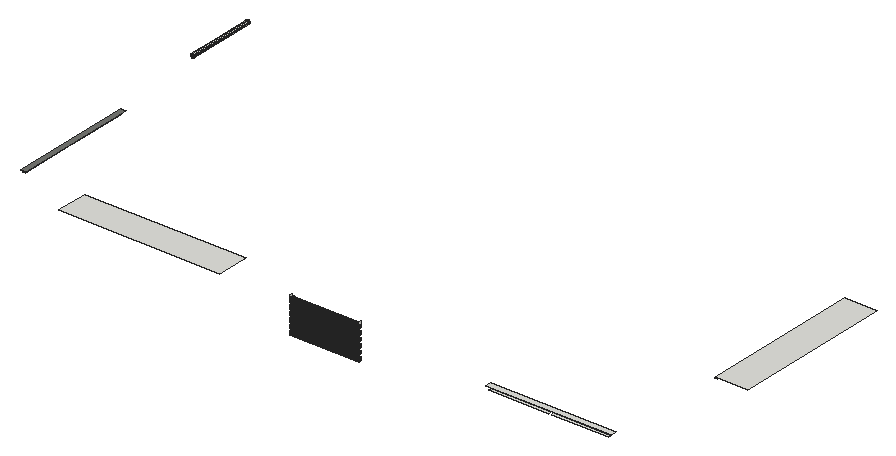
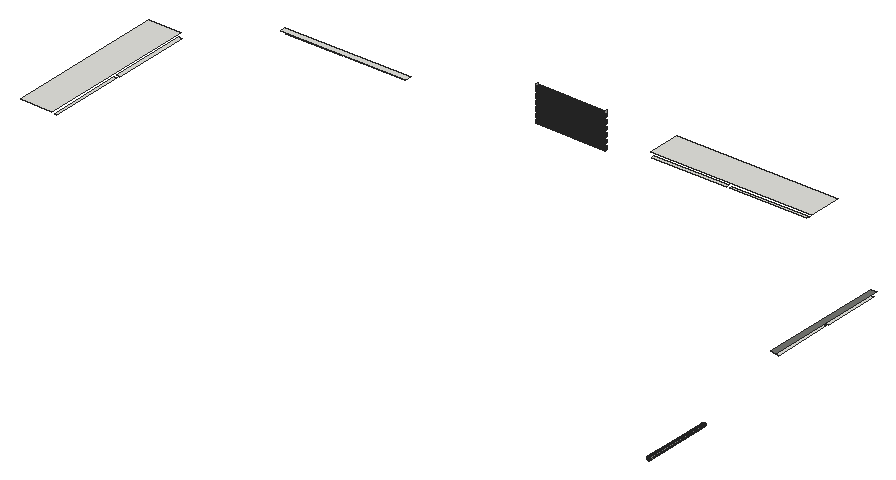
# SketchUp Ruby script. Lengths in inches.
U = 1.inch
M = Sketchup.active_model
def pt(a) = Geom::Point3d.new(a.map { |v| v * U })
def face(e, loops, mat)
  f = e.add_face(loops[0].map { |a| pt(a) })
  loops[1..].each { |l| e.add_face(l.map { |a| pt(a) }).erase! }
  f.material = f.back_material = mat if mat
  f
end
# faces: each face lists its corners as indices into pts; further lists are holes
def faces(e, pts, list, mat = nil) = list.each { |f| face(e, (f[0].is_a?(Array) ? f : [f]).map { |l| l.map { |i| pts[i] } }, mat) }
# xy, xz, yz: faces in a plane at the given z, y or x. An outline is a flat list of corners, or four numbers for a rectangle; further outlines are holes
def ring(l) = l.size == 4 ? [[l[0], l[1]], [l[2], l[1]], [l[2], l[3]], [l[0], l[3]]] : l.each_slice(2).to_a
def flat(e, list, mat, &to3) = list.each { |f| face(e, (f[0].is_a?(Array) ? f : [f]).map { |l| ring(l).map { |u, v| to3.(u, v) } }, mat) }
def xy(e, z, list, mat = nil) = flat(e, list, mat) { |x, y| [x, y, z] }
def xz(e, y, list, mat = nil) = flat(e, list, mat) { |x, z| [x, y, z] }
def yz(e, x, list, mat = nil) = flat(e, list, mat) { |y, z| [x, y, z] }
def lines(e, pts, list) = list.each { |a, b| e.add_line(pt(pts[a]), pt(pts[b])) }
# prism: a flat outline (further loops are holes) pulled along v
def prism(e, loops, v, mat = nil)
  f = face(e, loops, mat); d = Geom::Vector3d.new(v.map { |x| x * U })
  f.pushpull(f.normal.samedirection?(d) ? d.length : -d.length)
end
def box(e, o, s, mat = nil) = prism(e, [[o, [o[0] + s[0], o[1], o[2]], [o[0] + s[0], o[1] + s[1], o[2]], [o[0], o[1] + s[1], o[2]]]], [0, 0, s[2]], mat)
def at(x, y, z, deg = 0) = Geom::Transformation.translation(pt([x, y, z])) * Geom::Transformation.rotation(ORIGIN, Z_AXIS, deg.degrees)
def axes(o, x, y, z) = Geom::Transformation.new([*x, 0, *y, 0, *z, 0, *pt(o).to_a, 1])
def part(name) = M.definitions.add(name)
# library, detail: a bought-in or finely detailed component or shape, given as its bounding box
def library(name, o, s) = part(name).tap { |d| box(d.entities, o, s) }
def detail(e, o, s) = box(e.add_group.entities, o, s)
def put(e, d, t, mat = nil) = e.add_instance(d, t).tap { |i| i.material = mat if mat }
def group(e, t, mat = nil) = e.add_group.tap { |g| g.transformation = t; g.material = mat if mat }.entities
root = M.entities
M.materials.add("[Metal Seamed]").color = [118, 119, 115]
xy(root,647.61,[[1161.2,84.8125,1285.04,90.8125],[1291.04,84.8125,1408.89,90.8125],[120,175.92,126,293.77],[120,299.77,126,423.61]])
xy(root,653.61,[[1155.2,84.8125,1414.89,96.8125]])
xy(root,653.61,[[120,169.92,132,429.61]],"[Metal Seamed]")
xy(root,696.625,[[312.65,102.8125,473.9375,108.8125],[479.9375,102.8125,635.22,108.8125],[1476,277.47,1482,438.75],[1476,444.75,1482,600.03]])
xy(root,702.625,[[306.65,36.8125,641.22,102.8125],[1482,271.47,1548,606.03]])
yz(root,778.64,[[48.34,702.02,49.29,702.14,50.18,702.51,50.95,703.1,51.53,703.86,51.9,704.75,52.03,705.7,51.9,706.66,51.8,706.89,44.875,706.89,44.78,706.66,44.65,705.7,44.78,704.75,45.15,703.86,45.73,703.1,46.5,702.51,47.38,702.14]])
yz(root,922.01,[[48.34,702.02,47.38,702.14,46.5,702.51,45.73,703.1,45.15,703.86,44.78,704.75,44.65,705.7,44.78,706.66,44.875,706.89,51.8,706.89,51.9,706.66,52.03,705.7,51.9,704.75,51.53,703.86,50.95,703.1,50.18,702.51,49.29,702.14]])
p = [[922.01,48.34,633.02],[922.01,47.38,633.14],[778.64,47.38,633.14],[778.64,48.34,633.02],[922.01,49.29,633.14],[778.64,49.29,633.14],
  [83.53,662.8,633.02],[82.57,662.8,633.14],[82.57,806.17,633.14],[83.53,806.17,633.02],[84.48,662.8,633.14],[84.48,806.17,633.14],
  [922.01,46.5,633.51],[778.64,46.5,633.51],[922.01,50.18,633.51],[778.64,50.18,633.51],[81.68,662.8,633.51],[81.68,806.17,633.51],
  [85.37,662.8,633.51],[85.37,806.17,633.51],[922.01,45.73,634.1],[778.64,45.73,634.1],[922.01,50.95,634.1],[778.64,50.95,634.1],
  [80.92,662.8,634.1],[80.92,806.17,634.1],[86.13,662.8,634.1],[86.13,806.17,634.1],[922.01,45.15,634.86],[778.64,45.15,634.86],
  [922.01,51.53,634.86],[778.64,51.53,634.86],[80.33,662.8,634.86],[80.33,806.17,634.86],[86.72,662.8,634.86],[86.72,806.17,634.86],
  [922.01,44.78,635.75],[778.64,44.78,635.75],[922.01,51.9,635.75],[778.64,51.9,635.75],[79.97,662.8,635.75],[79.97,806.17,635.75],
  [87.09,662.8,635.75],[87.09,806.17,635.75],[922.01,44.65,636.7],[778.64,44.65,636.7],[922.01,52.03,636.7],[778.64,52.03,636.7],
  [79.84,662.8,636.7],[79.84,806.17,636.7],[87.21,662.8,636.7],[87.21,806.17,636.7],[922.01,44.78,637.66],[778.64,44.78,637.66],
  [922.01,51.9,637.66],[778.64,51.9,637.66],[79.97,662.8,637.66],[79.97,806.17,637.66],[87.09,662.8,637.66],[87.09,806.17,637.66],
  [922.01,45.15,638.55],[778.64,45.15,638.55],[922.01,51.53,638.55],[778.64,51.53,638.55],[80.33,662.8,638.55],[80.33,806.17,638.55],
  [86.72,662.8,638.55],[86.72,806.17,638.55],[922.01,45.73,639.3125],[778.64,45.73,639.3125],[922.01,50.95,639.3125],[778.64,50.95,639.3125],
  [80.92,662.8,639.3125],[80.92,806.17,639.3125],[86.13,662.8,639.3125],[86.13,806.17,639.3125],[922.01,46.5,639.9],[778.64,46.5,639.9],
  [922.01,50.18,639.9],[778.64,50.18,639.9],[81.68,662.8,639.9],[81.68,806.17,639.9],[85.37,662.8,639.9],[85.37,806.17,639.9],
  [922.01,47.38,640.27],[778.64,47.38,640.27],[922.01,49.29,640.27],[778.64,49.29,640.27],[82.57,662.8,640.27],[82.57,806.17,640.27],
  [84.48,662.8,640.27],[84.48,806.17,640.27],[922.01,48.34,640.39],[778.64,48.34,640.39],[83.53,662.8,640.39],[83.53,806.17,640.39],
  [922.01,48.34,645.02],[922.01,47.38,645.14],[778.64,47.38,645.14],[778.64,48.34,645.02],[922.01,49.29,645.14],[778.64,49.29,645.14],
  [922.01,46.5,645.51],[778.64,46.5,645.51],[922.01,50.18,645.51],[778.64,50.18,645.51],[922.01,45.73,646.1],[778.64,45.73,646.1],
  [922.01,50.95,646.1],[778.64,50.95,646.1],[922.01,45.15,646.86],[778.64,45.15,646.86],[922.01,51.53,646.86],[778.64,51.53,646.86],
  [922.01,44.78,647.75],[778.64,44.78,647.75],[922.01,51.9,647.75],[778.64,51.9,647.75],[922.01,44.65,648.7],[778.64,44.65,648.7],
  [922.01,52.03,648.7],[778.64,52.03,648.7],[922.01,44.78,649.66],[778.64,44.78,649.66],[922.01,51.9,649.66],[778.64,51.9,649.66],
  [922.01,45.15,650.55],[778.64,45.15,650.55],[922.01,51.53,650.55],[778.64,51.53,650.55],[922.01,45.73,651.3125],[778.64,45.73,651.3125],
  [922.01,50.95,651.3125],[778.64,50.95,651.3125],[922.01,46.5,651.9],[778.64,46.5,651.9],[922.01,50.18,651.9],[778.64,50.18,651.9],
  [922.01,47.38,652.27],[778.64,47.38,652.27],[922.01,49.29,652.27],[778.64,49.29,652.27],[922.01,48.34,652.39],[778.64,48.34,652.39],
  [922.01,48.34,657.02],[922.01,47.38,657.14],[778.64,47.38,657.14],[778.64,48.34,657.02],[922.01,49.29,657.14],[778.64,49.29,657.14],
  [922.01,46.5,657.51],[778.64,46.5,657.51],[922.01,50.18,657.51],[778.64,50.18,657.51],[922.01,45.73,658.1],[778.64,45.73,658.1],
  [922.01,50.95,658.1],[778.64,50.95,658.1],[922.01,45.15,658.86],[778.64,45.15,658.86],[922.01,51.53,658.86],[778.64,51.53,658.86],
  [922.01,44.78,659.75],[778.64,44.78,659.75],[922.01,51.9,659.75],[778.64,51.9,659.75],[922.01,44.65,660.7],[778.64,44.65,660.7],
  [922.01,52.03,660.7],[778.64,52.03,660.7],[922.01,44.78,661.66],[778.64,44.78,661.66],[922.01,51.9,661.66],[778.64,51.9,661.66],
  [922.01,45.15,662.55],[778.64,45.15,662.55],[922.01,51.53,662.55],[778.64,51.53,662.55],[922.01,45.73,663.3125],[778.64,45.73,663.3125],
  [922.01,50.95,663.3125],[778.64,50.95,663.3125],[922.01,46.5,663.9],[778.64,46.5,663.9],[922.01,50.18,663.9],[778.64,50.18,663.9],
  [922.01,47.38,664.27],[778.64,47.38,664.27],[922.01,49.29,664.27],[778.64,49.29,664.27],[922.01,48.34,664.39],[778.64,48.34,664.39],
  [922.01,48.34,669.02],[922.01,47.38,669.14],[778.64,47.38,669.14],[778.64,48.34,669.02],[922.01,49.29,669.14],[778.64,49.29,669.14],
  [922.01,46.5,669.51],[778.64,46.5,669.51],[922.01,50.18,669.51],[778.64,50.18,669.51],[922.01,45.73,670.1],[778.64,45.73,670.1],
  [922.01,50.95,670.1],[778.64,50.95,670.1],[922.01,45.15,670.86],[778.64,45.15,670.86],[922.01,51.53,670.86],[778.64,51.53,670.86],
  [922.01,44.78,671.75],[778.64,44.78,671.75],[922.01,51.9,671.75],[778.64,51.9,671.75],[922.01,44.65,672.7],[778.64,44.65,672.7],
  [922.01,52.03,672.7],[778.64,52.03,672.7],[922.01,44.78,673.66],[778.64,44.78,673.66],[922.01,51.9,673.66],[778.64,51.9,673.66],
  [922.01,45.15,674.55],[778.64,45.15,674.55],[922.01,51.53,674.55],[778.64,51.53,674.55],[922.01,45.73,675.3125],[778.64,45.73,675.3125],
  [922.01,50.95,675.3125],[778.64,50.95,675.3125],[922.01,46.5,675.9],[778.64,46.5,675.9],[922.01,50.18,675.9],[778.64,50.18,675.9],
  [922.01,47.38,676.27],[778.64,47.38,676.27],[922.01,49.29,676.27],[778.64,49.29,676.27],[922.01,48.34,676.39],[778.64,48.34,676.39],
  [922.01,48.34,681.02],[922.01,47.38,681.14],[778.64,47.38,681.14],[778.64,48.34,681.02],[922.01,49.29,681.14],[778.64,49.29,681.14],
  [922.01,46.5,681.51],[778.64,46.5,681.51],[922.01,50.18,681.51],[778.64,50.18,681.51],[922.01,45.73,682.1],[778.64,45.73,682.1],
  [922.01,50.95,682.1],[778.64,50.95,682.1],[922.01,45.15,682.86],[778.64,45.15,682.86],[922.01,51.53,682.86],[778.64,51.53,682.86],
  [922.01,44.78,683.75],[778.64,44.78,683.75],[922.01,51.9,683.75],[778.64,51.9,683.75],[922.01,44.65,684.7],[778.64,44.65,684.7],
  [922.01,52.03,684.7],[778.64,52.03,684.7],[922.01,44.78,685.66],[778.64,44.78,685.66],[922.01,51.9,685.66],[778.64,51.9,685.66],
  [922.01,45.15,686.55],[778.64,45.15,686.55],[922.01,51.53,686.55],[778.64,51.53,686.55],[922.01,45.73,687.3125],[778.64,45.73,687.3125],
  [922.01,50.95,687.3125],[778.64,50.95,687.3125],[922.01,46.5,687.9],[778.64,46.5,687.9],[922.01,50.18,687.9],[778.64,50.18,687.9],
  [922.01,47.38,688.27],[778.64,47.38,688.27],[922.01,49.29,688.27],[778.64,49.29,688.27],[922.01,48.34,688.39],[778.64,48.34,688.39],
  [922.01,48.34,693.02],[922.01,47.38,693.14],[778.64,47.38,693.14],[778.64,48.34,693.02],[922.01,49.29,693.14],[778.64,49.29,693.14],
  [922.01,46.5,693.51],[778.64,46.5,693.51],[922.01,50.18,693.51],[778.64,50.18,693.51],[922.01,45.73,694.1],[778.64,45.73,694.1],
  [922.01,50.95,694.1],[778.64,50.95,694.1],[922.01,45.15,694.86],[778.64,45.15,694.86],[922.01,51.53,694.86],[778.64,51.53,694.86],
  [922.01,44.78,695.75],[778.64,44.78,695.75],[922.01,51.9,695.75],[778.64,51.9,695.75],[922.01,44.65,696.7],[778.64,44.65,696.7],
  [922.01,52.03,696.7],[778.64,52.03,696.7],[922.01,44.78,697.66],[778.64,44.78,697.66],[922.01,51.9,697.66],[778.64,51.9,697.66],
  [922.01,45.15,698.55],[778.64,45.15,698.55],[922.01,51.53,698.55],[778.64,51.53,698.55],[922.01,45.73,699.3125],[778.64,45.73,699.3125],
  [922.01,50.95,699.3125],[778.64,50.95,699.3125],[922.01,46.5,699.9],[778.64,46.5,699.9],[922.01,50.18,699.9],[778.64,50.18,699.9],
  [922.01,47.38,700.27],[778.64,47.38,700.27],[922.01,49.29,700.27],[778.64,49.29,700.27],[922.01,48.34,700.39],[778.64,48.34,700.39],
  [922.01,48.34,702.02],[922.01,47.38,702.14],[778.64,47.38,702.14],[778.64,48.34,702.02],[922.01,49.29,702.14],[778.64,49.29,702.14],
  [922.01,46.5,702.51],[778.64,46.5,702.51],[922.01,50.18,702.51],[778.64,50.18,702.51],[922.01,45.73,703.1],[778.64,45.73,703.1],
  [922.01,50.95,703.1],[778.64,50.95,703.1],[922.01,45.15,703.86],[778.64,45.15,703.86],[922.01,51.53,703.86],[778.64,51.53,703.86]]
faces(root,p,[[0,1,2,3],[4,0,3,5],[6,7,8,9],[10,6,9,11],[1,12,13,2],[14,4,5,15],[7,16,17,8],[18,10,11,19],
  [12,20,21,13],[22,14,15,23],[16,24,25,17],[26,18,19,27],[20,28,29,21],[30,22,23,31],[24,32,33,25],[34,26,27,35],
  [28,36,37,29],[38,30,31,39],[32,40,41,33],[42,34,35,43],[36,44,45,37],[46,38,39,47],[40,48,49,41],[50,42,43,51],
  [44,52,53,45],[54,46,47,55],[48,56,57,49],[58,50,51,59],[52,60,61,53],[62,54,55,63],[56,64,65,57],[66,58,59,67],
  [60,68,69,61],[70,62,63,71],[64,72,73,65],[74,66,67,75],[68,76,77,69],[78,70,71,79],[72,80,81,73],[82,74,75,83],
  [76,84,85,77],[86,78,79,87],[80,88,89,81],[90,82,83,91],[84,92,93,85],[92,86,87,93],[88,94,95,89],[94,90,91,95],
  [96,97,98,99],[100,96,99,101],[97,102,103,98],[104,100,101,105],[102,106,107,103],[108,104,105,109],[106,110,111,107],[112,108,109,113],
  [110,114,115,111],[116,112,113,117],[114,118,119,115],[120,116,117,121],[118,122,123,119],[124,120,121,125],[122,126,127,123],[128,124,125,129],
  [126,130,131,127],[132,128,129,133],[130,134,135,131],[136,132,133,137],[134,138,139,135],[140,136,137,141],[138,142,143,139],[142,140,141,143],
  [144,145,146,147],[148,144,147,149],[145,150,151,146],[152,148,149,153],[150,154,155,151],[156,152,153,157],[154,158,159,155],[160,156,157,161],
  [158,162,163,159],[164,160,161,165],[162,166,167,163],[168,164,165,169],[166,170,171,167],[172,168,169,173],[170,174,175,171],[176,172,173,177],
  [174,178,179,175],[180,176,177,181],[178,182,183,179],[184,180,181,185],[182,186,187,183],[188,184,185,189],[186,190,191,187],[190,188,189,191],
  [192,193,194,195],[196,192,195,197],[193,198,199,194],[200,196,197,201],[198,202,203,199],[204,200,201,205],[202,206,207,203],[208,204,205,209],
  [206,210,211,207],[212,208,209,213],[210,214,215,211],[216,212,213,217],[214,218,219,215],[220,216,217,221],[218,222,223,219],[224,220,221,225],
  [222,226,227,223],[228,224,225,229],[226,230,231,227],[232,228,229,233],[230,234,235,231],[236,232,233,237],[234,238,239,235],[238,236,237,239],
  [240,241,242,243],[244,240,243,245],[241,246,247,242],[248,244,245,249],[246,250,251,247],[252,248,249,253],[250,254,255,251],[256,252,253,257],
  [254,258,259,255],[260,256,257,261],[258,262,263,259],[264,260,261,265],[262,266,267,263],[268,264,265,269],[266,270,271,267],[272,268,269,273],
  [270,274,275,271],[276,272,273,277],[274,278,279,275],[280,276,277,281],[278,282,283,279],[284,280,281,285],[282,286,287,283],[286,284,285,287],
  [288,289,290,291],[292,288,291,293],[289,294,295,290],[296,292,293,297],[294,298,299,295],[300,296,297,301],[298,302,303,299],[304,300,301,305],
  [302,306,307,303],[308,304,305,309],[306,310,311,307],[312,308,309,313],[310,314,315,311],[316,312,313,317],[314,318,319,315],[320,316,317,321],
  [318,322,323,319],[324,320,321,325],[322,326,327,323],[328,324,325,329],[326,330,331,327],[332,328,329,333],[330,334,335,331],[334,332,333,335],
  [336,337,338,339],[340,336,339,341],[337,342,343,338],[344,340,341,345],[342,346,347,343],[348,344,345,349],[346,350,351,347],[352,348,349,353]])
